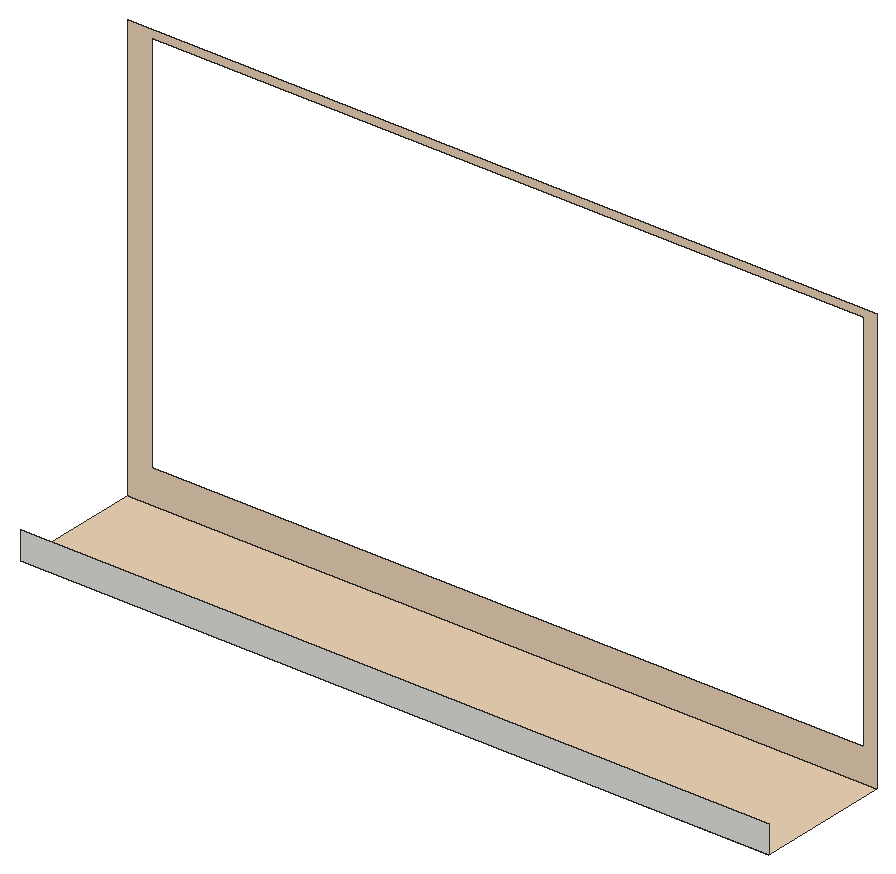
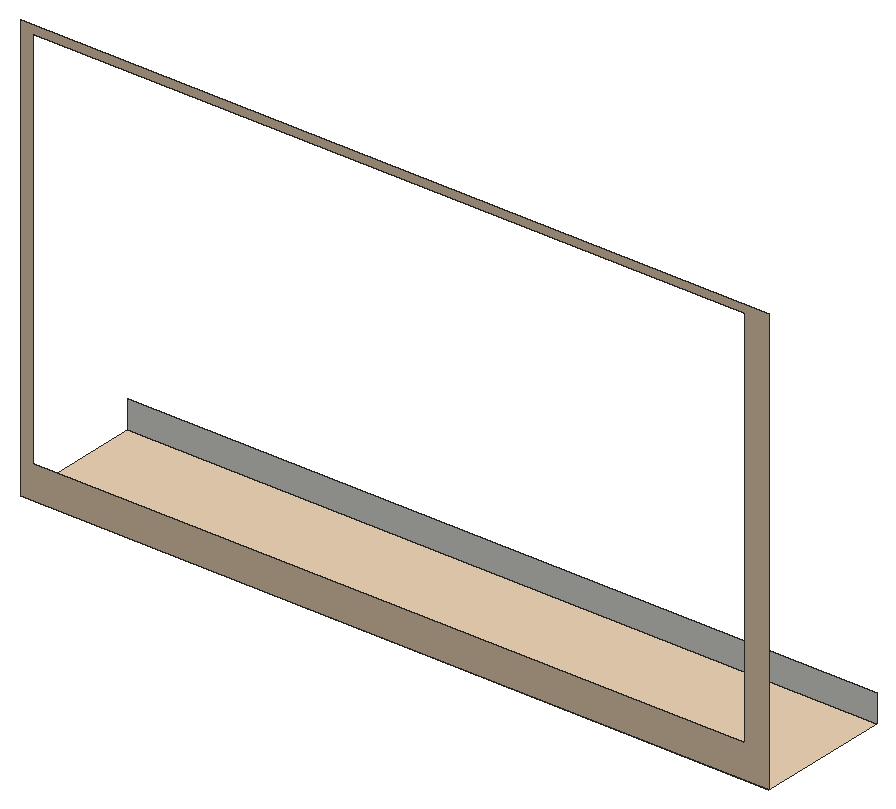
# SketchUp Ruby script. Lengths in inches.
U = 1.inch
M = Sketchup.active_model
def pt(a) = Geom::Point3d.new(a.map { |v| v * U })
def face(e, loops, mat)
  f = e.add_face(loops[0].map { |a| pt(a) })
  loops[1..].each { |l| e.add_face(l.map { |a| pt(a) }).erase! }
  f.material = f.back_material = mat if mat
  f
end
# faces: each face lists its corners as indices into pts; further lists are holes
def faces(e, pts, list, mat = nil) = list.each { |f| face(e, (f[0].is_a?(Array) ? f : [f]).map { |l| l.map { |i| pts[i] } }, mat) }
# xy, xz, yz: faces in a plane at the given z, y or x. An outline is a flat list of corners, or four numbers for a rectangle; further outlines are holes
def ring(l) = l.size == 4 ? [[l[0], l[1]], [l[2], l[1]], [l[2], l[3]], [l[0], l[3]]] : l.each_slice(2).to_a
def flat(e, list, mat, &to3) = list.each { |f| face(e, (f[0].is_a?(Array) ? f : [f]).map { |l| ring(l).map { |u, v| to3.(u, v) } }, mat) }
def xy(e, z, list, mat = nil) = flat(e, list, mat) { |x, y| [x, y, z] }
def xz(e, y, list, mat = nil) = flat(e, list, mat) { |x, z| [x, y, z] }
def yz(e, x, list, mat = nil) = flat(e, list, mat) { |y, z| [x, y, z] }
def lines(e, pts, list) = list.each { |a, b| e.add_line(pt(pts[a]), pt(pts[b])) }
# prism: a flat outline (further loops are holes) pulled along v
def prism(e, loops, v, mat = nil)
  f = face(e, loops, mat); d = Geom::Vector3d.new(v.map { |x| x * U })
  f.pushpull(f.normal.samedirection?(d) ? d.length : -d.length)
end
def box(e, o, s, mat = nil) = prism(e, [[o, [o[0] + s[0], o[1], o[2]], [o[0] + s[0], o[1] + s[1], o[2]], [o[0], o[1] + s[1], o[2]]]], [0, 0, s[2]], mat)
def at(x, y, z, deg = 0) = Geom::Transformation.translation(pt([x, y, z])) * Geom::Transformation.rotation(ORIGIN, Z_AXIS, deg.degrees)
def axes(o, x, y, z) = Geom::Transformation.new([*x, 0, *y, 0, *z, 0, *pt(o).to_a, 1])
def part(name) = M.definitions.add(name)
# library, detail: a bought-in or finely detailed component or shape, given as its bounding box
def library(name, o, s) = part(name).tap { |d| box(d.entities, o, s) }
def detail(e, o, s) = box(e.add_group.entities, o, s)
def put(e, d, t, mat = nil) = e.add_instance(d, t).tap { |i| i.material = mat if mat }
def group(e, t, mat = nil) = e.add_group.tap { |g| g.transformation = t; g.material = mat if mat }.entities
root = M.entities
M.materials.add("[0012_Bisque]1").color = [237, 212, 182]
xy(root,103.6875,[[211.5,374.19,376.86,403.76]],"[0012_Bisque]1")
xz(root,374.19,[[211.5,103.6875,376.86,109.8125]])
xz(root,403.76,[[[211.5,103.6875,376.86,197.75],[216.9,111.1,374.03,196.03]]],"[0012_Bisque]1")
